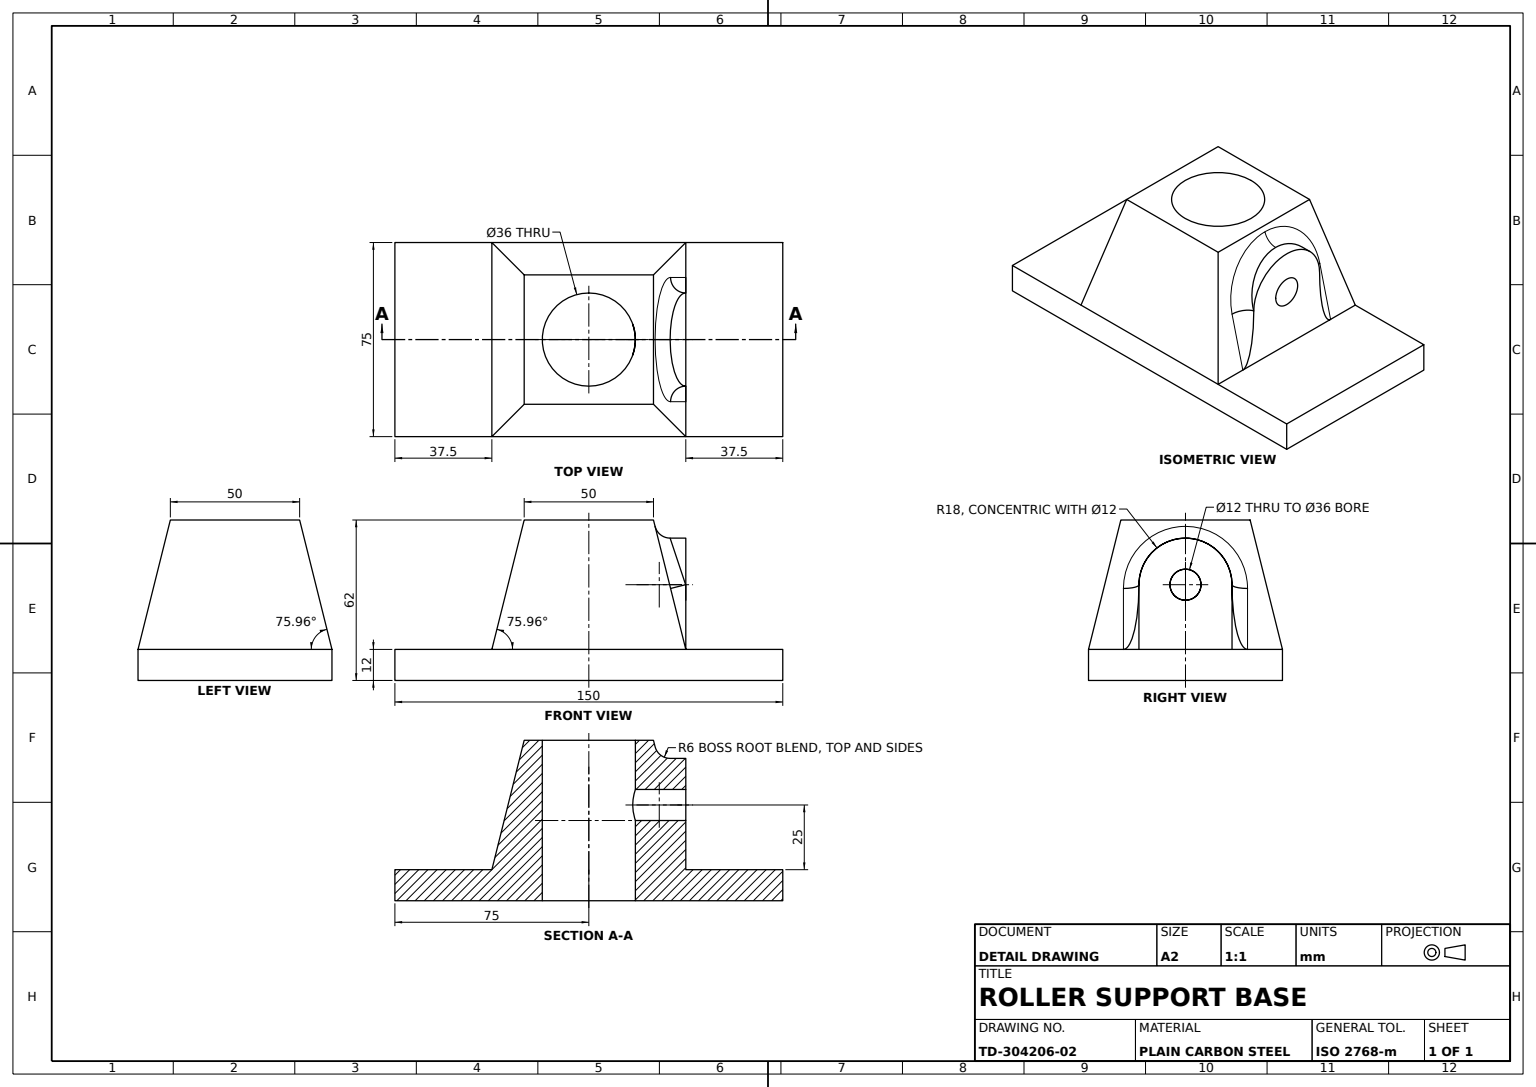
ISO-10303-21;
HEADER;
FILE_DESCRIPTION((''),'2;1');
FILE_NAME('','',(''),(''),'','','');
FILE_SCHEMA(('AUTOMOTIVE_DESIGN'));
ENDSEC;
DATA;
#1=APPLICATION_CONTEXT('');
#2=PRODUCT_CONTEXT('',#1,'mechanical');
#3=PRODUCT('','','',(#2));
#4=PRODUCT_DEFINITION_FORMATION('','',#3);
#5=PRODUCT_DEFINITION_CONTEXT('',#1,'design');
#6=PRODUCT_DEFINITION('','',#4,#5);
#7=PRODUCT_DEFINITION_SHAPE('','',#6);
#8=(LENGTH_UNIT()NAMED_UNIT(*)SI_UNIT(.MILLI.,.METRE.));
#9=(NAMED_UNIT(*)PLANE_ANGLE_UNIT()SI_UNIT($,.RADIAN.));
#10=(NAMED_UNIT(*)SI_UNIT($,.STERADIAN.)SOLID_ANGLE_UNIT());
#11=UNCERTAINTY_MEASURE_WITH_UNIT(LENGTH_MEASURE(1.E-05),#8,'distance_accuracy_value','');
#12=(GEOMETRIC_REPRESENTATION_CONTEXT(3)GLOBAL_UNCERTAINTY_ASSIGNED_CONTEXT((#11))GLOBAL_UNIT_ASSIGNED_CONTEXT((#8,#9,#10))REPRESENTATION_CONTEXT('',''));
#13=CARTESIAN_POINT('',(-37.5,12.,37.5));
#14=VERTEX_POINT('',#13);
#15=CARTESIAN_POINT('',(37.5,12.,37.5));
#16=VERTEX_POINT('',#15);
#17=DIRECTION('',(1.,0.,0.));
#18=VECTOR('',#17,1000.);
#19=LINE('',#13,#18);
#20=EDGE_CURVE('',#14,#16,#19,.T.);
#21=ORIENTED_EDGE('',*,*,#20,.F.);
#22=CARTESIAN_POINT('',(-75.,12.,37.5));
#23=VERTEX_POINT('',#22);
#24=LINE('',#22,#18);
#25=EDGE_CURVE('',#23,#14,#24,.T.);
#26=ORIENTED_EDGE('',*,*,#25,.F.);
#27=CARTESIAN_POINT('',(-75.,0.,37.5));
#28=VERTEX_POINT('',#27);
#29=DIRECTION('',(0.,-1.,0.));
#30=VECTOR('',#29,1000.);
#31=LINE('',#22,#30);
#32=EDGE_CURVE('',#23,#28,#31,.T.);
#33=ORIENTED_EDGE('',*,*,#32,.T.);
#34=CARTESIAN_POINT('',(75.,0.,37.5));
#35=VERTEX_POINT('',#34);
#36=LINE('',#27,#18);
#37=EDGE_CURVE('',#28,#35,#36,.T.);
#38=ORIENTED_EDGE('',*,*,#37,.T.);
#39=CARTESIAN_POINT('',(75.,12.,37.5));
#40=VERTEX_POINT('',#39);
#41=LINE('',#39,#30);
#42=EDGE_CURVE('',#40,#35,#41,.T.);
#43=ORIENTED_EDGE('',*,*,#42,.F.);
#44=EDGE_CURVE('',#16,#40,#24,.T.);
#45=ORIENTED_EDGE('',*,*,#44,.F.);
#46=EDGE_LOOP('',(#21,#26,#33,#38,#43,#45));
#47=FACE_OUTER_BOUND('',#46,.T.);
#48=DIRECTION('',(0.,0.,-1.));
#49=DIRECTION('',(-1.,0.,0.));
#50=AXIS2_PLACEMENT_3D('',#22,#48,#49);
#51=PLANE('',#50);
#52=ADVANCED_FACE('',(#47),#51,.F.);
#53=CARTESIAN_POINT('',(0.,0.,-18.));
#54=VERTEX_POINT('',#53);
#55=CARTESIAN_POINT('',(0.,62.,-18.));
#56=VERTEX_POINT('',#55);
#57=DIRECTION('',(0.,1.,0.));
#58=VECTOR('',#57,1000.);
#59=LINE('',#53,#58);
#60=EDGE_CURVE('',#54,#56,#59,.T.);
#61=ORIENTED_EDGE('',*,*,#60,.F.);
#62=CARTESIAN_POINT('',(0.,0.,18.));
#63=VERTEX_POINT('',#62);
#64=CARTESIAN_POINT('',(0.,0.,0.));
#65=DIRECTION('',(0.,0.,1.));
#66=AXIS2_PLACEMENT_3D('',#64,#57,#65);
#67=CIRCLE('',#66,18.);
#68=EDGE_CURVE('',#63,#54,#67,.T.);
#69=ORIENTED_EDGE('',*,*,#68,.F.);
#70=CARTESIAN_POINT('',(0.,62.,18.));
#71=VERTEX_POINT('',#70);
#72=LINE('',#62,#58);
#73=EDGE_CURVE('',#63,#71,#72,.T.);
#74=ORIENTED_EDGE('',*,*,#73,.T.);
#75=CARTESIAN_POINT('',(0.,62.,0.));
#76=AXIS2_PLACEMENT_3D('',#75,#57,#65);
#77=CIRCLE('',#76,18.);
#78=EDGE_CURVE('',#71,#56,#77,.T.);
#79=ORIENTED_EDGE('',*,*,#78,.T.);
#80=EDGE_LOOP('',(#61,#69,#74,#79));
#81=FACE_OUTER_BOUND('',#80,.T.);
#82=CARTESIAN_POINT('',(16.970563,37.,6.));
#83=VERTEX_POINT('',#82);
#84=CARTESIAN_POINT('',(16.970563,37.,-6.));
#85=VERTEX_POINT('',#84);
#86=CARTESIAN_POINT('',(16.970563,37.196707,6.));
#87=CARTESIAN_POINT('',(16.973984,37.393341,5.99035));
#88=CARTESIAN_POINT('',(16.987641,37.786461,5.951512));
#89=CARTESIAN_POINT('',(16.997961,37.984057,5.922079));
#90=CARTESIAN_POINT('',(17.038406,38.567807,5.805128));
#91=CARTESIAN_POINT('',(17.077659,38.942932,5.690221));
#92=CARTESIAN_POINT('',(17.17505,39.666628,5.389127));
#93=CARTESIAN_POINT('',(17.233783,40.017317,5.200744));
#94=CARTESIAN_POINT('',(17.358867,40.664856,4.766631));
#95=CARTESIAN_POINT('',(17.42558,40.965236,4.520005));
#96=CARTESIAN_POINT('',(17.526382,41.380881,4.10442));
#97=CARTESIAN_POINT('',(17.560044,41.513248,3.958362));
#98=CARTESIAN_POINT('',(17.625288,41.760781,3.656911));
#99=CARTESIAN_POINT('',(17.657049,41.876696,3.500803));
#100=CARTESIAN_POINT('',(17.718026,42.093056,3.177824));
#101=CARTESIAN_POINT('',(17.747243,42.193501,3.010954));
#102=CARTESIAN_POINT('',(17.80231,42.378666,2.66613));
#103=CARTESIAN_POINT('',(17.828282,42.463775,2.487203));
#104=CARTESIAN_POINT('',(17.898918,42.691404,1.940099));
#105=CARTESIAN_POINT('',(17.93598,42.805575,1.565128));
#106=CARTESIAN_POINT('',(17.973936,42.921461,0.987362));
#107=CARTESIAN_POINT('',(17.983648,42.950793,0.792204));
#108=CARTESIAN_POINT('',(17.99672,42.990182,0.396543));
#109=CARTESIAN_POINT('',(18.00001,43.000029,0.196786));
#110=CARTESIAN_POINT('',(17.999981,42.999942,-0.396219));
#111=CARTESIAN_POINT('',(17.986952,42.961191,-0.787767));
#112=CARTESIAN_POINT('',(17.948883,42.844976,-1.369433));
#113=CARTESIAN_POINT('',(17.93299,42.796128,-1.563305));
#114=CARTESIAN_POINT('',(17.89603,42.680746,-1.941173));
#115=CARTESIAN_POINT('',(17.874948,42.614166,-2.125896));
#116=CARTESIAN_POINT('',(17.804921,42.388474,-2.667871));
#117=CARTESIAN_POINT('',(17.748824,42.202395,-3.014912));
#118=CARTESIAN_POINT('',(17.625429,41.764439,-3.668068));
#119=CARTESIAN_POINT('',(17.559435,41.51718,-3.968159));
#120=CARTESIAN_POINT('',(17.426063,40.967219,-4.518005));
#121=CARTESIAN_POINT('',(17.358028,40.660914,-4.769676));
#122=CARTESIAN_POINT('',(17.232961,40.012655,-5.203462));
#123=CARTESIAN_POINT('',(17.175524,39.66976,-5.387632));
#124=CARTESIAN_POINT('',(17.102274,39.126038,-5.614135));
#125=CARTESIAN_POINT('',(17.079907,38.938715,-5.68159));
#126=CARTESIAN_POINT('',(17.041123,38.560526,-5.796882));
#127=CARTESIAN_POINT('',(17.02466,38.369658,-5.84488));
#128=CARTESIAN_POINT('',(16.984677,37.791796,-5.960487));
#129=CARTESIAN_POINT('',(16.970563,37.399442,-6.));
#130=B_SPLINE_CURVE_WITH_KNOTS('',3,(#82,#86,#87,#88,#89,#90,#91,#92,#93,#94,#95,#96,#97,#98,#99,#100,#101,#102,#103,#104,#105,#106,#107,#108,#109,#110,#111,#112,#113,#114,#115,#116,#117,#118,#119,#120,#121,#122,#123,#124,#125,#126,#127,#128,#129,#84),.UNSPECIFIED.,.F.,.F.,(4,2,2,2,2,2,2,2,2,2,2,2,2,2,2,2,2,2,2,2,2,2,4),(0.018894458,0.019484755,0.020075052,0.021255646,0.02243624,0.023616834,0.024207132,0.024797429,0.025387726,0.025978023,0.027158617,0.027748914,0.028339211,0.029519805,0.030110103,0.0307004,0.031880994,0.033061588,0.034242182,0.035422777,0.036013074,0.036603371,0.037783965),.UNSPECIFIED.);
#131=EDGE_CURVE('',#83,#85,#130,.T.);
#132=ORIENTED_EDGE('',*,*,#131,.F.);
#133=CARTESIAN_POINT('',(16.970563,36.600454,-6.));
#134=CARTESIAN_POINT('',(16.984674,36.208204,-5.960495));
#135=CARTESIAN_POINT('',(17.024673,35.630173,-5.844843));
#136=CARTESIAN_POINT('',(17.041144,35.439232,-5.79682));
#137=CARTESIAN_POINT('',(17.079955,35.06086,-5.681448));
#138=CARTESIAN_POINT('',(17.10231,34.873676,-5.614028));
#139=CARTESIAN_POINT('',(17.175582,34.329856,-5.387447));
#140=CARTESIAN_POINT('',(17.233108,33.986414,-5.203008));
#141=CARTESIAN_POINT('',(17.327208,33.498923,-4.876546));
#142=CARTESIAN_POINT('',(17.360054,33.340323,-4.758683));
#143=CARTESIAN_POINT('',(17.426295,33.037993,-4.510078));
#144=CARTESIAN_POINT('',(17.459739,32.893881,-4.379212));
#145=CARTESIAN_POINT('',(17.559641,32.482042,-3.967226));
#146=CARTESIAN_POINT('',(17.625686,32.23459,-3.666928));
#147=CARTESIAN_POINT('',(17.749388,31.795664,-3.011707));
#148=CARTESIAN_POINT('',(17.805,31.61127,-2.667235));
#149=CARTESIAN_POINT('',(17.874886,31.386031,-2.126379));
#150=CARTESIAN_POINT('',(17.895938,31.319544,-1.941992));
#151=CARTESIAN_POINT('',(17.932865,31.204258,-1.564699));
#152=CARTESIAN_POINT('',(17.948782,31.155335,-1.370779));
#153=CARTESIAN_POINT('',(17.986914,31.038921,-0.788748));
#154=CARTESIAN_POINT('',(17.99994,31.000181,-0.397405));
#155=CARTESIAN_POINT('',(18.00006,30.99982,0.391911));
#156=CARTESIAN_POINT('',(17.986698,31.039576,0.7927));
#157=CARTESIAN_POINT('',(17.936027,31.19428,1.564811));
#158=CARTESIAN_POINT('',(17.898891,31.308676,1.940441));
#159=CARTESIAN_POINT('',(17.804555,31.612696,2.670849));
#160=CARTESIAN_POINT('',(17.748407,31.799112,3.017028));
#161=CARTESIAN_POINT('',(17.656751,32.124378,3.502318));
#162=CARTESIAN_POINT('',(17.6249,32.240646,3.658804));
#163=CARTESIAN_POINT('',(17.559415,32.489187,3.96117));
#164=CARTESIAN_POINT('',(17.525676,32.621954,4.107414));
#165=CARTESIAN_POINT('',(17.425195,33.036501,4.521419));
#166=CARTESIAN_POINT('',(17.358573,33.336511,4.7677));
#167=CARTESIAN_POINT('',(17.233449,33.984567,5.201854));
#168=CARTESIAN_POINT('',(17.174736,34.335494,5.390115));
#169=CARTESIAN_POINT('',(17.077603,35.057694,5.690376));
#170=CARTESIAN_POINT('',(17.038443,35.432012,5.80502));
#171=CARTESIAN_POINT('',(16.998052,36.014459,5.921817));
#172=CARTESIAN_POINT('',(16.98768,36.2126,5.951399));
#173=CARTESIAN_POINT('',(16.973986,36.60641,5.990345));
#174=CARTESIAN_POINT('',(16.970563,36.803242,6.));
#175=B_SPLINE_CURVE_WITH_KNOTS('',3,(#84,#133,#134,#135,#136,#137,#138,#139,#140,#141,#142,#143,#144,#145,#146,#147,#148,#149,#150,#151,#152,#153,#154,#155,#156,#157,#158,#159,#160,#161,#162,#163,#164,#165,#166,#167,#168,#169,#170,#171,#172,#173,#174,#82),.UNSPECIFIED.,.F.,.F.,(4,2,2,2,2,2,2,2,2,2,2,2,2,2,2,2,2,2,2,2,2,4),(0.,0.001180904,0.001771355,0.002361807,0.003542711,0.004133163,0.004723614,0.005904518,0.007085422,0.007675873,0.008266325,0.009447229,0.010628132,0.011809036,0.01298994,0.013580391,0.014170843,0.015351747,0.01653265,0.017713554,0.018304006,0.018894458),.UNSPECIFIED.);
#176=EDGE_CURVE('',#85,#83,#175,.T.);
#177=ORIENTED_EDGE('',*,*,#176,.F.);
#178=EDGE_LOOP('',(#132,#177));
#179=FACE_BOUND('',#178,.T.);
#180=CYLINDRICAL_SURFACE('',#66,18.);
#181=ADVANCED_FACE('',(#81,#179),#180,.F.);
#182=EDGE_CURVE('',#54,#63,#67,.T.);
#183=ORIENTED_EDGE('',*,*,#182,.T.);
#184=ORIENTED_EDGE('',*,*,#68,.T.);
#185=EDGE_LOOP('',(#183,#184));
#186=FACE_BOUND('',#185,.T.);
#187=ORIENTED_EDGE('',*,*,#37,.F.);
#188=CARTESIAN_POINT('',(-75.,0.,-37.5));
#189=VERTEX_POINT('',#188);
#190=VECTOR('',#65,1000.);
#191=LINE('',#27,#190);
#192=EDGE_CURVE('',#189,#28,#191,.T.);
#193=ORIENTED_EDGE('',*,*,#192,.F.);
#194=CARTESIAN_POINT('',(75.,0.,-37.5));
#195=VERTEX_POINT('',#194);
#196=VECTOR('',#49,1000.);
#197=LINE('',#188,#196);
#198=EDGE_CURVE('',#195,#189,#197,.T.);
#199=ORIENTED_EDGE('',*,*,#198,.F.);
#200=VECTOR('',#48,1000.);
#201=LINE('',#34,#200);
#202=EDGE_CURVE('',#35,#195,#201,.T.);
#203=ORIENTED_EDGE('',*,*,#202,.F.);
#204=EDGE_LOOP('',(#187,#193,#199,#203));
#205=FACE_OUTER_BOUND('',#204,.T.);
#206=AXIS2_PLACEMENT_3D('',#64,#29,#48);
#207=PLANE('',#206);
#208=ADVANCED_FACE('',(#186,#205),#207,.T.);
#209=ORIENTED_EDGE('',*,*,#176,.T.);
#210=CARTESIAN_POINT('',(37.5,37.,6.));
#211=VERTEX_POINT('',#210);
#212=CARTESIAN_POINT('',(-75.001025,37.,6.));
#213=LINE('',#212,#18);
#214=EDGE_CURVE('',#83,#211,#213,.T.);
#215=ORIENTED_EDGE('',*,*,#214,.T.);
#216=CARTESIAN_POINT('',(37.5,37.,-6.));
#217=VERTEX_POINT('',#216);
#218=CARTESIAN_POINT('',(37.5,37.,0.));
#219=AXIS2_PLACEMENT_3D('',#218,#17,#48);
#220=CIRCLE('',#219,6.);
#221=EDGE_CURVE('',#211,#217,#220,.T.);
#222=ORIENTED_EDGE('',*,*,#221,.T.);
#223=CARTESIAN_POINT('',(-75.001025,37.,-6.));
#224=LINE('',#223,#18);
#225=EDGE_CURVE('',#85,#217,#224,.T.);
#226=ORIENTED_EDGE('',*,*,#225,.F.);
#227=EDGE_LOOP('',(#209,#215,#222,#226));
#228=FACE_OUTER_BOUND('',#227,.T.);
#229=CARTESIAN_POINT('',(-75.001025,37.,0.));
#230=AXIS2_PLACEMENT_3D('',#229,#17,#48);
#231=CYLINDRICAL_SURFACE('',#230,6.);
#232=ADVANCED_FACE('',(#228),#231,.F.);
#233=CARTESIAN_POINT('',(37.5,12.,-37.5));
#234=VERTEX_POINT('',#233);
#235=CARTESIAN_POINT('',(-37.5,12.,-37.5));
#236=VERTEX_POINT('',#235);
#237=LINE('',#235,#196);
#238=EDGE_CURVE('',#234,#236,#237,.T.);
#239=ORIENTED_EDGE('',*,*,#238,.F.);
#240=CARTESIAN_POINT('',(75.,12.,-37.5));
#241=VERTEX_POINT('',#240);
#242=CARTESIAN_POINT('',(-75.,12.,-37.5));
#243=LINE('',#242,#196);
#244=EDGE_CURVE('',#241,#234,#243,.T.);
#245=ORIENTED_EDGE('',*,*,#244,.F.);
#246=LINE('',#240,#30);
#247=EDGE_CURVE('',#241,#195,#246,.T.);
#248=ORIENTED_EDGE('',*,*,#247,.T.);
#249=ORIENTED_EDGE('',*,*,#198,.T.);
#250=VERTEX_POINT('',#242);
#251=LINE('',#242,#30);
#252=EDGE_CURVE('',#250,#189,#251,.T.);
#253=ORIENTED_EDGE('',*,*,#252,.F.);
#254=EDGE_CURVE('',#236,#250,#243,.T.);
#255=ORIENTED_EDGE('',*,*,#254,.F.);
#256=EDGE_LOOP('',(#239,#245,#248,#249,#253,#255));
#257=FACE_OUTER_BOUND('',#256,.T.);
#258=AXIS2_PLACEMENT_3D('',#242,#65,#17);
#259=PLANE('',#258);
#260=ADVANCED_FACE('',(#257),#259,.F.);
#261=ORIENTED_EDGE('',*,*,#254,.T.);
#262=LINE('',#22,#190);
#263=EDGE_CURVE('',#250,#23,#262,.T.);
#264=ORIENTED_EDGE('',*,*,#263,.T.);
#265=ORIENTED_EDGE('',*,*,#25,.T.);
#266=LINE('',#13,#190);
#267=EDGE_CURVE('',#236,#14,#266,.T.);
#268=ORIENTED_EDGE('',*,*,#267,.F.);
#269=EDGE_LOOP('',(#261,#264,#265,#268));
#270=FACE_OUTER_BOUND('',#269,.T.);
#271=CARTESIAN_POINT('',(0.,12.,0.));
#272=AXIS2_PLACEMENT_3D('',#271,#29,#48);
#273=PLANE('',#272);
#274=ADVANCED_FACE('',(#270),#273,.F.);
#275=CARTESIAN_POINT('',(31.613803,35.544786,-24.));
#276=VERTEX_POINT('',#275);
#277=CARTESIAN_POINT('',(37.5,12.,-24.));
#278=VERTEX_POINT('',#277);
#279=CARTESIAN_POINT('',(38.117647,9.529412,-24.));
#280=DIRECTION('',(0.242535625,-0.9701425,0.));
#281=VECTOR('',#280,1000.);
#282=LINE('',#279,#281);
#283=EDGE_CURVE('',#276,#278,#282,.T.);
#284=ORIENTED_EDGE('',*,*,#283,.F.);
#285=CARTESIAN_POINT('',(37.434658,37.,-18.));
#286=VERTEX_POINT('',#285);
#287=CARTESIAN_POINT('',(37.434658,37.,-24.));
#288=DIRECTION('',(0.9701425,0.242535625,0.));
#289=AXIS2_PLACEMENT_3D('',#287,#280,#288);
#290=CIRCLE('',#289,6.);
#291=EDGE_CURVE('',#286,#276,#290,.T.);
#292=ORIENTED_EDGE('',*,*,#291,.F.);
#293=CARTESIAN_POINT('',(37.5,36.738634,-18.));
#294=VERTEX_POINT('',#293);
#295=CARTESIAN_POINT('',(43.320855,13.455214,-18.));
#296=DIRECTION('',(-0.242535625,0.9701425,0.));
#297=VECTOR('',#296,1000.);
#298=LINE('',#295,#297);
#299=EDGE_CURVE('',#294,#286,#298,.T.);
#300=ORIENTED_EDGE('',*,*,#299,.F.);
#301=CARTESIAN_POINT('',(37.5,12.,-20.485281));
#302=CARTESIAN_POINT('',(37.5,22.247078,-18.));
#303=(BOUNDED_CURVE()B_SPLINE_CURVE(3,(#277,#301,#302,#293),.UNSPECIFIED.,.F.,.F.)B_SPLINE_CURVE_WITH_KNOTS((4,4),(0.,1.570796327),.UNSPECIFIED.)CURVE()GEOMETRIC_REPRESENTATION_ITEM()RATIONAL_B_SPLINE_CURVE((1.,0.804737854,0.804737854,1.))REPRESENTATION_ITEM(''));
#304=EDGE_CURVE('',#278,#294,#303,.T.);
#305=ORIENTED_EDGE('',*,*,#304,.F.);
#306=EDGE_LOOP('',(#284,#292,#300,#305));
#307=FACE_OUTER_BOUND('',#306,.T.);
#308=CARTESIAN_POINT('',(43.938502,10.984626,-24.));
#309=AXIS2_PLACEMENT_3D('',#308,#280,#288);
#310=CYLINDRICAL_SURFACE('',#309,6.);
#311=ADVANCED_FACE('',(#307),#310,.F.);
#312=CARTESIAN_POINT('',(31.613803,35.544786,24.));
#313=VERTEX_POINT('',#312);
#314=CARTESIAN_POINT('',(25.613803,59.544786,0.));
#315=VERTEX_POINT('',#314);
#316=CARTESIAN_POINT('',(28.099085,49.603661,24.));
#317=CARTESIAN_POINT('',(25.613803,59.544786,14.058875));
#318=(BOUNDED_CURVE()B_SPLINE_CURVE(3,(#312,#316,#317,#314),.UNSPECIFIED.,.F.,.F.)B_SPLINE_CURVE_WITH_KNOTS((4,4),(4.71238898,6.283185307),.UNSPECIFIED.)CURVE()GEOMETRIC_REPRESENTATION_ITEM()RATIONAL_B_SPLINE_CURVE((1.,0.804737854,0.804737854,1.))REPRESENTATION_ITEM(''));
#319=EDGE_CURVE('',#313,#315,#318,.T.);
#320=ORIENTED_EDGE('',*,*,#319,.T.);
#321=CARTESIAN_POINT('',(25.613803,59.544786,-14.058875));
#322=CARTESIAN_POINT('',(28.099085,49.603661,-24.));
#323=(BOUNDED_CURVE()B_SPLINE_CURVE(3,(#314,#321,#322,#275),.UNSPECIFIED.,.F.,.F.)B_SPLINE_CURVE_WITH_KNOTS((4,4),(0.,1.570796327),.UNSPECIFIED.)CURVE()GEOMETRIC_REPRESENTATION_ITEM()RATIONAL_B_SPLINE_CURVE((1.,0.804737854,0.804737854,1.))REPRESENTATION_ITEM(''));
#324=EDGE_CURVE('',#315,#276,#323,.T.);
#325=ORIENTED_EDGE('',*,*,#324,.T.);
#326=ORIENTED_EDGE('',*,*,#283,.T.);
#327=LINE('',#15,#200);
#328=EDGE_CURVE('',#278,#234,#327,.T.);
#329=ORIENTED_EDGE('',*,*,#328,.T.);
#330=CARTESIAN_POINT('',(25.,62.,-25.));
#331=VERTEX_POINT('',#330);
#332=DIRECTION('',(0.23570226,-0.942809042,-0.23570226));
#333=VECTOR('',#332,1000.);
#334=LINE('',#330,#333);
#335=EDGE_CURVE('',#331,#234,#334,.T.);
#336=ORIENTED_EDGE('',*,*,#335,.F.);
#337=CARTESIAN_POINT('',(25.,62.,25.));
#338=VERTEX_POINT('',#337);
#339=LINE('',#337,#200);
#340=EDGE_CURVE('',#338,#331,#339,.T.);
#341=ORIENTED_EDGE('',*,*,#340,.F.);
#342=DIRECTION('',(0.23570226,-0.942809042,0.23570226));
#343=VECTOR('',#342,1000.);
#344=LINE('',#337,#343);
#345=EDGE_CURVE('',#338,#16,#344,.T.);
#346=ORIENTED_EDGE('',*,*,#345,.T.);
#347=CARTESIAN_POINT('',(37.5,12.,24.));
#348=VERTEX_POINT('',#347);
#349=EDGE_CURVE('',#16,#348,#327,.T.);
#350=ORIENTED_EDGE('',*,*,#349,.T.);
#351=CARTESIAN_POINT('',(38.117647,9.529412,24.));
#352=LINE('',#351,#297);
#353=EDGE_CURVE('',#348,#313,#352,.T.);
#354=ORIENTED_EDGE('',*,*,#353,.T.);
#355=EDGE_LOOP('',(#320,#325,#326,#329,#336,#341,#346,#350,#354));
#356=FACE_OUTER_BOUND('',#355,.T.);
#357=CARTESIAN_POINT('',(38.117647,9.529412,0.));
#358=AXIS2_PLACEMENT_3D('',#357,#288,#296);
#359=PLANE('',#358);
#360=ADVANCED_FACE('',(#356),#359,.T.);
#361=ORIENTED_EDGE('',*,*,#299,.T.);
#362=CARTESIAN_POINT('',(37.5,37.,-18.));
#363=VERTEX_POINT('',#362);
#364=LINE('',#362,#196);
#365=EDGE_CURVE('',#363,#286,#364,.T.);
#366=ORIENTED_EDGE('',*,*,#365,.F.);
#367=CARTESIAN_POINT('',(37.5,12.,-18.));
#368=LINE('',#367,#58);
#369=EDGE_CURVE('',#294,#363,#368,.T.);
#370=ORIENTED_EDGE('',*,*,#369,.F.);
#371=EDGE_LOOP('',(#361,#366,#370));
#372=FACE_OUTER_BOUND('',#371,.T.);
#373=AXIS2_PLACEMENT_3D('',#367,#65,#29);
#374=PLANE('',#373);
#375=ADVANCED_FACE('',(#372),#374,.F.);
#376=ORIENTED_EDGE('',*,*,#32,.F.);
#377=ORIENTED_EDGE('',*,*,#263,.F.);
#378=ORIENTED_EDGE('',*,*,#252,.T.);
#379=ORIENTED_EDGE('',*,*,#192,.T.);
#380=EDGE_LOOP('',(#376,#377,#378,#379));
#381=FACE_OUTER_BOUND('',#380,.T.);
#382=AXIS2_PLACEMENT_3D('',#22,#17,#48);
#383=PLANE('',#382);
#384=ADVANCED_FACE('',(#381),#383,.F.);
#385=ORIENTED_EDGE('',*,*,#345,.F.);
#386=CARTESIAN_POINT('',(-25.,62.,25.));
#387=VERTEX_POINT('',#386);
#388=LINE('',#386,#18);
#389=EDGE_CURVE('',#387,#338,#388,.T.);
#390=ORIENTED_EDGE('',*,*,#389,.F.);
#391=DIRECTION('',(-0.23570226,-0.942809042,0.23570226));
#392=VECTOR('',#391,1000.);
#393=LINE('',#386,#392);
#394=EDGE_CURVE('',#387,#14,#393,.T.);
#395=ORIENTED_EDGE('',*,*,#394,.T.);
#396=ORIENTED_EDGE('',*,*,#20,.T.);
#397=EDGE_LOOP('',(#385,#390,#395,#396));
#398=FACE_OUTER_BOUND('',#397,.T.);
#399=CARTESIAN_POINT('',(0.,9.529412,38.117647));
#400=DIRECTION('',(0.,0.242535625,0.9701425));
#401=DIRECTION('',(0.,-0.9701425,0.242535625));
#402=AXIS2_PLACEMENT_3D('',#399,#400,#401);
#403=PLANE('',#402);
#404=ADVANCED_FACE('',(#398),#403,.T.);
#405=ORIENTED_EDGE('',*,*,#353,.F.);
#406=CARTESIAN_POINT('',(37.5,36.738634,18.));
#407=VERTEX_POINT('',#406);
#408=CARTESIAN_POINT('',(37.5,22.247078,18.));
#409=CARTESIAN_POINT('',(37.5,12.,20.485281));
#410=(BOUNDED_CURVE()B_SPLINE_CURVE(3,(#406,#408,#409,#347),.UNSPECIFIED.,.F.,.T.)B_SPLINE_CURVE_WITH_KNOTS((4,4),(1.570796327,3.141592654),.UNSPECIFIED.)CURVE()GEOMETRIC_REPRESENTATION_ITEM()RATIONAL_B_SPLINE_CURVE((1.,0.804737854,0.804737854,1.))REPRESENTATION_ITEM(''));
#411=EDGE_CURVE('',#407,#348,#410,.T.);
#412=ORIENTED_EDGE('',*,*,#411,.F.);
#413=CARTESIAN_POINT('',(37.434658,37.,18.));
#414=VERTEX_POINT('',#413);
#415=CARTESIAN_POINT('',(37.438502,36.984626,18.));
#416=LINE('',#415,#281);
#417=EDGE_CURVE('',#414,#407,#416,.T.);
#418=ORIENTED_EDGE('',*,*,#417,.F.);
#419=CARTESIAN_POINT('',(37.434658,37.,24.));
#420=DIRECTION('',(-0.9701425,-0.242535625,0.));
#421=AXIS2_PLACEMENT_3D('',#419,#296,#420);
#422=CIRCLE('',#421,6.);
#423=EDGE_CURVE('',#414,#313,#422,.T.);
#424=ORIENTED_EDGE('',*,*,#423,.T.);
#425=EDGE_LOOP('',(#405,#412,#418,#424));
#426=FACE_OUTER_BOUND('',#425,.T.);
#427=CARTESIAN_POINT('',(43.938502,10.984626,24.));
#428=AXIS2_PLACEMENT_3D('',#427,#296,#420);
#429=CYLINDRICAL_SURFACE('',#428,6.);
#430=ADVANCED_FACE('',(#426),#429,.F.);
#431=ORIENTED_EDGE('',*,*,#182,.F.);
#432=ORIENTED_EDGE('',*,*,#60,.T.);
#433=EDGE_CURVE('',#56,#71,#77,.T.);
#434=ORIENTED_EDGE('',*,*,#433,.T.);
#435=ORIENTED_EDGE('',*,*,#73,.F.);
#436=EDGE_LOOP('',(#431,#432,#434,#435));
#437=FACE_OUTER_BOUND('',#436,.T.);
#438=ADVANCED_FACE('',(#437),#180,.F.);
#439=ORIENTED_EDGE('',*,*,#42,.T.);
#440=ORIENTED_EDGE('',*,*,#202,.T.);
#441=ORIENTED_EDGE('',*,*,#247,.F.);
#442=LINE('',#39,#200);
#443=EDGE_CURVE('',#40,#241,#442,.T.);
#444=ORIENTED_EDGE('',*,*,#443,.F.);
#445=EDGE_LOOP('',(#439,#440,#441,#444));
#446=FACE_OUTER_BOUND('',#445,.T.);
#447=AXIS2_PLACEMENT_3D('',#39,#49,#65);
#448=PLANE('',#447);
#449=ADVANCED_FACE('',(#446),#448,.F.);
#450=ORIENTED_EDGE('',*,*,#423,.F.);
#451=CARTESIAN_POINT('',(31.434658,55.,0.));
#452=VERTEX_POINT('',#451);
#453=CARTESIAN_POINT('',(31.434658,55.,10.544156));
#454=CARTESIAN_POINT('',(33.91994,47.544156,18.));
#455=(BOUNDED_CURVE()B_SPLINE_CURVE(3,(#451,#453,#454,#413),.UNSPECIFIED.,.F.,.F.)B_SPLINE_CURVE_WITH_KNOTS((4,4),(0.,1.570796327),.UNSPECIFIED.)CURVE()GEOMETRIC_REPRESENTATION_ITEM()RATIONAL_B_SPLINE_CURVE((1.,0.804737854,0.804737854,1.))REPRESENTATION_ITEM(''));
#456=EDGE_CURVE('',#452,#414,#455,.T.);
#457=ORIENTED_EDGE('',*,*,#456,.F.);
#458=CARTESIAN_POINT('',(31.434658,61.,0.));
#459=AXIS2_PLACEMENT_3D('',#458,#48,#49);
#460=CIRCLE('',#459,6.);
#461=EDGE_CURVE('',#452,#315,#460,.T.);
#462=ORIENTED_EDGE('',*,*,#461,.T.);
#463=ORIENTED_EDGE('',*,*,#319,.F.);
#464=EDGE_LOOP('',(#450,#457,#462,#463));
#465=FACE_OUTER_BOUND('',#464,.T.);
#466=CARTESIAN_POINT('',(26.75,55.,0.));
#467=CARTESIAN_POINT('',(31.434658,55.,1.178111));
#468=CARTESIAN_POINT('',(26.75,55.,1.25477));
#469=CARTESIAN_POINT('',(25.613803,59.544786,1.570814));
#470=CARTESIAN_POINT('',(31.473335,54.88397,2.356165));
#471=CARTESIAN_POINT('',(26.782885,54.86846,2.510988));
#472=CARTESIAN_POINT('',(25.65248,59.39008,3.141554));
#473=CARTESIAN_POINT('',(31.626559,54.4243,4.667086));
#474=CARTESIAN_POINT('',(26.912581,54.349676,4.965206));
#475=CARTESIAN_POINT('',(25.805704,58.777186,6.222782));
#476=CARTESIAN_POINT('',(31.741102,54.08067,5.799882));
#477=CARTESIAN_POINT('',(27.0097,53.961199,6.165927));
#478=CARTESIAN_POINT('',(25.920247,58.319013,7.733176));
#479=CARTESIAN_POINT('',(32.041661,53.178993,7.976722));
#480=CARTESIAN_POINT('',(27.263063,52.94775,8.45699));
#481=CARTESIAN_POINT('',(26.220806,57.116777,10.635629));
#482=CARTESIAN_POINT('',(32.227669,52.620969,9.020712));
#483=CARTESIAN_POINT('',(27.419879,52.320482,9.549392));
#484=CARTESIAN_POINT('',(26.406814,56.372745,12.027616));
#485=CARTESIAN_POINT('',(32.664013,51.311937,10.979816));
#486=CARTESIAN_POINT('',(27.785127,50.859491,11.577398));
#487=CARTESIAN_POINT('',(26.843158,54.627369,14.639755));
#488=CARTESIAN_POINT('',(32.914338,50.560963,11.894882));
#489=CARTESIAN_POINT('',(27.994316,50.022736,12.514021));
#490=CARTESIAN_POINT('',(27.093483,53.62607,15.859842));
#491=CARTESIAN_POINT('',(33.469698,48.894882,13.560963));
#492=CARTESIAN_POINT('',(28.454473,48.182109,14.192043));
#493=CARTESIAN_POINT('',(27.648843,51.404628,18.081283));
#494=CARTESIAN_POINT('',(33.77472,47.979816,14.311937));
#495=CARTESIAN_POINT('',(28.706271,47.174915,14.933204));
#496=CARTESIAN_POINT('',(27.953865,50.184541,19.082583));
#497=CARTESIAN_POINT('',(34.427754,46.020712,15.620969));
#498=CARTESIAN_POINT('',(29.239994,45.040025,16.191818));
#499=CARTESIAN_POINT('',(28.606899,47.572402,20.827958));
#500=CARTESIAN_POINT('',(34.775751,44.976722,16.178993));
#501=CARTESIAN_POINT('',(29.522693,43.909226,16.707738));
#502=CARTESIAN_POINT('',(28.954896,46.180415,21.571991));
#503=CARTESIAN_POINT('',(35.501364,42.799882,17.08067));
#504=CARTESIAN_POINT('',(30.10537,41.57852,17.498831));
#505=CARTESIAN_POINT('',(29.680509,43.277962,22.774227));
#506=CARTESIAN_POINT('',(35.878963,41.667086,17.4243));
#507=CARTESIAN_POINT('',(30.405939,40.376243,17.771334));
#508=CARTESIAN_POINT('',(30.058108,41.767568,23.2324));
#509=CARTESIAN_POINT('',(36.64927,39.356165,17.88397));
#510=CARTESIAN_POINT('',(31.011038,37.955847,18.070889));
#511=CARTESIAN_POINT('',(30.828415,38.68634,23.845294));
#512=CARTESIAN_POINT('',(37.041955,38.178111,18.));
#513=CARTESIAN_POINT('',(31.315876,36.736496,18.094491));
#514=CARTESIAN_POINT('',(31.2211,37.1156,24.));
#515=CARTESIAN_POINT('',(31.613803,35.544786,18.));
#516=(BOUNDED_SURFACE()B_SPLINE_SURFACE(3,2,((#451,#466,#314),(#467,#468,#469),(#470,#471,#472),(#473,#474,#475),(#476,#477,#478),(#479,#480,#481),(#482,#483,#484),(#485,#486,#487),(#488,#489,#490),(#491,#492,#493),(#494,#495,#496),(#497,#498,#499),(#500,#501,#502),(#503,#504,#505),(#506,#507,#508),(#509,#510,#511),(#512,#513,#514),(#413,#515,#312)),.UNSPECIFIED.,.F.,.F.,.T.)B_SPLINE_SURFACE_WITH_KNOTS((4,2,2,2,2,2,2,2,4),(3,3),(0.,0.196349541,0.392699082,0.589048623,0.785398163,0.981747704,1.178097245,1.374446786,1.570796327),(0.,1.),.UNSPECIFIED.)GEOMETRIC_REPRESENTATION_ITEM()RATIONAL_B_SPLINE_SURFACE(((1.,0.788205438,1.),(1.,0.78820586,1.),(1.,0.787710022,1.),(1.,0.785741834,1.),(1.,0.784269062,1.),(1.,0.780386619,1.),(1.,0.777976947,1.),(1.,0.772288193,1.),(1.,0.769009112,1.),(1.,0.761676085,1.),(1.,0.757622147,1.),(1.,0.748860892,1.),(1.,0.744153599,1.),(1.,0.734233607,1.),(1.,0.72902096,1.),(1.,0.718263638,1.),(1.,0.712719396,1.),(1.,0.707106781,1.)))REPRESENTATION_ITEM('')SURFACE());
#517=ADVANCED_FACE('',(#465),#516,.F.);
#518=CARTESIAN_POINT('',(33.91994,47.544156,-18.));
#519=CARTESIAN_POINT('',(31.434658,55.,-10.544156));
#520=(BOUNDED_CURVE()B_SPLINE_CURVE(3,(#285,#518,#519,#451),.UNSPECIFIED.,.F.,.F.)B_SPLINE_CURVE_WITH_KNOTS((4,4),(4.71238898,6.283185307),.UNSPECIFIED.)CURVE()GEOMETRIC_REPRESENTATION_ITEM()RATIONAL_B_SPLINE_CURVE((1.,0.804737854,0.804737854,1.))REPRESENTATION_ITEM(''));
#521=EDGE_CURVE('',#286,#452,#520,.T.);
#522=ORIENTED_EDGE('',*,*,#521,.F.);
#523=ORIENTED_EDGE('',*,*,#291,.T.);
#524=ORIENTED_EDGE('',*,*,#324,.F.);
#525=ORIENTED_EDGE('',*,*,#461,.F.);
#526=EDGE_LOOP('',(#522,#523,#524,#525));
#527=FACE_OUTER_BOUND('',#526,.T.);
#528=CARTESIAN_POINT('',(31.613803,35.544786,-18.));
#529=CARTESIAN_POINT('',(37.041955,38.178111,-18.));
#530=CARTESIAN_POINT('',(31.315876,36.736496,-18.094491));
#531=CARTESIAN_POINT('',(31.2211,37.1156,-24.));
#532=CARTESIAN_POINT('',(36.64927,39.356165,-17.88397));
#533=CARTESIAN_POINT('',(31.011038,37.955847,-18.070889));
#534=CARTESIAN_POINT('',(30.828415,38.68634,-23.845294));
#535=CARTESIAN_POINT('',(35.878963,41.667086,-17.4243));
#536=CARTESIAN_POINT('',(30.405939,40.376243,-17.771334));
#537=CARTESIAN_POINT('',(30.058108,41.767568,-23.2324));
#538=CARTESIAN_POINT('',(35.501364,42.799882,-17.08067));
#539=CARTESIAN_POINT('',(30.10537,41.57852,-17.498831));
#540=CARTESIAN_POINT('',(29.680509,43.277962,-22.774227));
#541=CARTESIAN_POINT('',(34.775751,44.976722,-16.178993));
#542=CARTESIAN_POINT('',(29.522693,43.909226,-16.707738));
#543=CARTESIAN_POINT('',(28.954896,46.180415,-21.571991));
#544=CARTESIAN_POINT('',(34.427754,46.020712,-15.620969));
#545=CARTESIAN_POINT('',(29.239994,45.040025,-16.191818));
#546=CARTESIAN_POINT('',(28.606899,47.572402,-20.827958));
#547=CARTESIAN_POINT('',(33.77472,47.979816,-14.311937));
#548=CARTESIAN_POINT('',(28.706271,47.174915,-14.933204));
#549=CARTESIAN_POINT('',(27.953865,50.184541,-19.082583));
#550=CARTESIAN_POINT('',(33.469698,48.894882,-13.560963));
#551=CARTESIAN_POINT('',(28.454473,48.182109,-14.192043));
#552=CARTESIAN_POINT('',(27.648843,51.404628,-18.081283));
#553=CARTESIAN_POINT('',(32.914338,50.560963,-11.894882));
#554=CARTESIAN_POINT('',(27.994316,50.022736,-12.514021));
#555=CARTESIAN_POINT('',(27.093483,53.62607,-15.859842));
#556=CARTESIAN_POINT('',(32.664013,51.311937,-10.979816));
#557=CARTESIAN_POINT('',(27.785127,50.859491,-11.577398));
#558=CARTESIAN_POINT('',(26.843158,54.627369,-14.639755));
#559=CARTESIAN_POINT('',(32.227669,52.620969,-9.020712));
#560=CARTESIAN_POINT('',(27.419879,52.320482,-9.549392));
#561=CARTESIAN_POINT('',(26.406814,56.372745,-12.027616));
#562=CARTESIAN_POINT('',(32.041661,53.178993,-7.976722));
#563=CARTESIAN_POINT('',(27.263063,52.94775,-8.45699));
#564=CARTESIAN_POINT('',(26.220806,57.116777,-10.635629));
#565=CARTESIAN_POINT('',(31.741102,54.08067,-5.799882));
#566=CARTESIAN_POINT('',(27.0097,53.961199,-6.165927));
#567=CARTESIAN_POINT('',(25.920247,58.319013,-7.733176));
#568=CARTESIAN_POINT('',(31.626559,54.4243,-4.667086));
#569=CARTESIAN_POINT('',(26.912581,54.349676,-4.965206));
#570=CARTESIAN_POINT('',(25.805704,58.777186,-6.222782));
#571=CARTESIAN_POINT('',(31.473335,54.88397,-2.356165));
#572=CARTESIAN_POINT('',(26.782885,54.86846,-2.510988));
#573=CARTESIAN_POINT('',(25.65248,59.39008,-3.141554));
#574=CARTESIAN_POINT('',(31.434658,55.,-1.178111));
#575=CARTESIAN_POINT('',(26.75,55.,-1.25477));
#576=CARTESIAN_POINT('',(25.613803,59.544786,-1.570814));
#577=(BOUNDED_SURFACE()B_SPLINE_SURFACE(3,2,((#285,#528,#275),(#529,#530,#531),(#532,#533,#534),(#535,#536,#537),(#538,#539,#540),(#541,#542,#543),(#544,#545,#546),(#547,#548,#549),(#550,#551,#552),(#553,#554,#555),(#556,#557,#558),(#559,#560,#561),(#562,#563,#564),(#565,#566,#567),(#568,#569,#570),(#571,#572,#573),(#574,#575,#576),(#451,#466,#314)),.UNSPECIFIED.,.F.,.F.,.F.)B_SPLINE_SURFACE_WITH_KNOTS((4,2,2,2,2,2,2,2,4),(3,3),(4.71238898,4.908738521,5.105088062,5.301437603,5.497787144,5.694136685,5.890486225,6.086835766,6.283185307),(0.,1.),.UNSPECIFIED.)GEOMETRIC_REPRESENTATION_ITEM()RATIONAL_B_SPLINE_SURFACE(((1.,0.707106781,1.),(1.,0.712719396,1.),(1.,0.718263638,1.),(1.,0.72902096,1.),(1.,0.734233607,1.),(1.,0.744153599,1.),(1.,0.748860892,1.),(1.,0.757622147,1.),(1.,0.761676085,1.),(1.,0.769009112,1.),(1.,0.772288193,1.),(1.,0.777976947,1.),(1.,0.780386619,1.),(1.,0.784269062,1.),(1.,0.785741834,1.),(1.,0.787710022,1.),(1.,0.78820586,1.),(1.,0.788205438,1.)))REPRESENTATION_ITEM('')SURFACE());
#578=ADVANCED_FACE('',(#527),#577,.F.);
#579=ORIENTED_EDGE('',*,*,#417,.T.);
#580=CARTESIAN_POINT('',(37.5,37.,18.));
#581=VERTEX_POINT('',#580);
#582=LINE('',#580,#30);
#583=EDGE_CURVE('',#581,#407,#582,.T.);
#584=ORIENTED_EDGE('',*,*,#583,.F.);
#585=LINE('',#580,#196);
#586=EDGE_CURVE('',#581,#414,#585,.T.);
#587=ORIENTED_EDGE('',*,*,#586,.T.);
#588=EDGE_LOOP('',(#579,#584,#587));
#589=FACE_OUTER_BOUND('',#588,.T.);
#590=AXIS2_PLACEMENT_3D('',#580,#48,#49);
#591=PLANE('',#590);
#592=ADVANCED_FACE('',(#589),#591,.F.);
#593=ORIENTED_EDGE('',*,*,#394,.F.);
#594=CARTESIAN_POINT('',(-25.,62.,-25.));
#595=VERTEX_POINT('',#594);
#596=LINE('',#386,#190);
#597=EDGE_CURVE('',#595,#387,#596,.T.);
#598=ORIENTED_EDGE('',*,*,#597,.F.);
#599=DIRECTION('',(-0.23570226,-0.942809042,-0.23570226));
#600=VECTOR('',#599,1000.);
#601=LINE('',#594,#600);
#602=EDGE_CURVE('',#595,#236,#601,.T.);
#603=ORIENTED_EDGE('',*,*,#602,.T.);
#604=ORIENTED_EDGE('',*,*,#267,.T.);
#605=EDGE_LOOP('',(#593,#598,#603,#604));
#606=FACE_OUTER_BOUND('',#605,.T.);
#607=CARTESIAN_POINT('',(-38.117647,9.529412,0.));
#608=DIRECTION('',(-0.9701425,0.242535625,0.));
#609=DIRECTION('',(-0.242535625,-0.9701425,0.));
#610=AXIS2_PLACEMENT_3D('',#607,#608,#609);
#611=PLANE('',#610);
#612=ADVANCED_FACE('',(#606),#611,.T.);
#613=ORIENTED_EDGE('',*,*,#521,.T.);
#614=ORIENTED_EDGE('',*,*,#456,.T.);
#615=ORIENTED_EDGE('',*,*,#586,.F.);
#616=CIRCLE('',#219,18.);
#617=EDGE_CURVE('',#363,#581,#616,.T.);
#618=ORIENTED_EDGE('',*,*,#617,.F.);
#619=ORIENTED_EDGE('',*,*,#365,.T.);
#620=EDGE_LOOP('',(#613,#614,#615,#618,#619));
#621=FACE_OUTER_BOUND('',#620,.T.);
#622=AXIS2_PLACEMENT_3D('',#218,#49,#65);
#623=CYLINDRICAL_SURFACE('',#622,18.);
#624=ADVANCED_FACE('',(#621),#623,.T.);
#625=ORIENTED_EDGE('',*,*,#602,.F.);
#626=LINE('',#594,#196);
#627=EDGE_CURVE('',#331,#595,#626,.T.);
#628=ORIENTED_EDGE('',*,*,#627,.F.);
#629=ORIENTED_EDGE('',*,*,#335,.T.);
#630=ORIENTED_EDGE('',*,*,#238,.T.);
#631=EDGE_LOOP('',(#625,#628,#629,#630));
#632=FACE_OUTER_BOUND('',#631,.T.);
#633=CARTESIAN_POINT('',(0.,9.529412,-38.117647));
#634=DIRECTION('',(0.,0.242535625,-0.9701425));
#635=DIRECTION('',(0.,0.9701425,0.242535625));
#636=AXIS2_PLACEMENT_3D('',#633,#634,#635);
#637=PLANE('',#636);
#638=ADVANCED_FACE('',(#632),#637,.T.);
#639=CARTESIAN_POINT('',(37.5,12.,18.));
#640=LINE('',#639,#200);
#641=EDGE_CURVE('',#348,#278,#640,.T.);
#642=ORIENTED_EDGE('',*,*,#641,.F.);
#643=ORIENTED_EDGE('',*,*,#349,.F.);
#644=ORIENTED_EDGE('',*,*,#44,.T.);
#645=ORIENTED_EDGE('',*,*,#443,.T.);
#646=ORIENTED_EDGE('',*,*,#244,.T.);
#647=ORIENTED_EDGE('',*,*,#328,.F.);
#648=EDGE_LOOP('',(#642,#643,#644,#645,#646,#647));
#649=FACE_OUTER_BOUND('',#648,.T.);
#650=ADVANCED_FACE('',(#649),#273,.F.);
#651=ORIENTED_EDGE('',*,*,#597,.T.);
#652=ORIENTED_EDGE('',*,*,#389,.T.);
#653=ORIENTED_EDGE('',*,*,#340,.T.);
#654=ORIENTED_EDGE('',*,*,#627,.T.);
#655=EDGE_LOOP('',(#651,#652,#653,#654));
#656=FACE_OUTER_BOUND('',#655,.T.);
#657=ORIENTED_EDGE('',*,*,#433,.F.);
#658=ORIENTED_EDGE('',*,*,#78,.F.);
#659=EDGE_LOOP('',(#657,#658));
#660=FACE_BOUND('',#659,.T.);
#661=AXIS2_PLACEMENT_3D('',#75,#29,#48);
#662=PLANE('',#661);
#663=ADVANCED_FACE('',(#656,#660),#662,.F.);
#664=ORIENTED_EDGE('',*,*,#221,.F.);
#665=EDGE_CURVE('',#217,#211,#220,.T.);
#666=ORIENTED_EDGE('',*,*,#665,.F.);
#667=EDGE_LOOP('',(#664,#666));
#668=FACE_BOUND('',#667,.T.);
#669=ORIENTED_EDGE('',*,*,#583,.T.);
#670=ORIENTED_EDGE('',*,*,#411,.T.);
#671=ORIENTED_EDGE('',*,*,#641,.T.);
#672=ORIENTED_EDGE('',*,*,#304,.T.);
#673=ORIENTED_EDGE('',*,*,#369,.T.);
#674=ORIENTED_EDGE('',*,*,#617,.T.);
#675=EDGE_LOOP('',(#669,#670,#671,#672,#673,#674));
#676=FACE_OUTER_BOUND('',#675,.T.);
#677=PLANE('',#219);
#678=ADVANCED_FACE('',(#668,#676),#677,.T.);
#679=ORIENTED_EDGE('',*,*,#131,.T.);
#680=ORIENTED_EDGE('',*,*,#225,.T.);
#681=ORIENTED_EDGE('',*,*,#665,.T.);
#682=ORIENTED_EDGE('',*,*,#214,.F.);
#683=EDGE_LOOP('',(#679,#680,#681,#682));
#684=FACE_OUTER_BOUND('',#683,.T.);
#685=ADVANCED_FACE('',(#684),#231,.F.);
#686=CLOSED_SHELL('',(#52,#181,#208,#232,#260,#274,#311,#360,#375,#384,#404,#430,#438,#449,#517,#578,#592,#612,#624,#638,#650,#663,#678,#685));
#687=MANIFOLD_SOLID_BREP('',#686);
#688=ADVANCED_BREP_SHAPE_REPRESENTATION('',(#687),#12);
#689=SHAPE_DEFINITION_REPRESENTATION(#7,#688);
ENDSEC;
END-ISO-10303-21;
